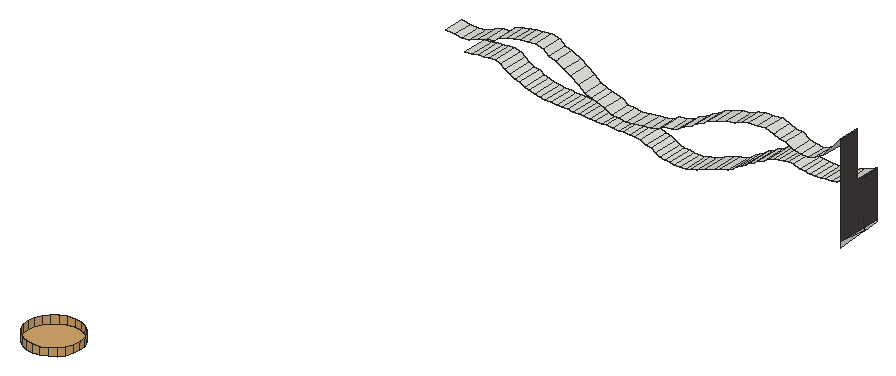
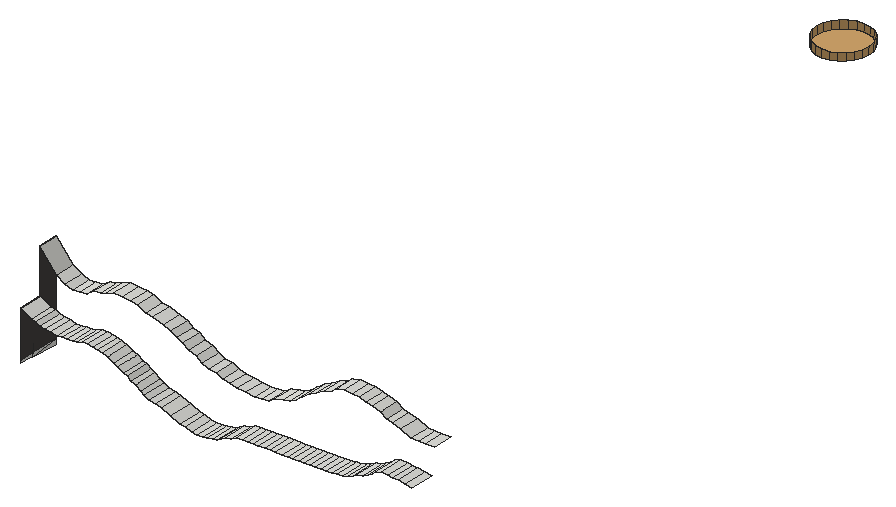
# SketchUp Ruby script. Lengths in inches.
U = 1.inch
M = Sketchup.active_model
def pt(a) = Geom::Point3d.new(a.map { |v| v * U })
def face(e, loops, mat)
  f = e.add_face(loops[0].map { |a| pt(a) })
  loops[1..].each { |l| e.add_face(l.map { |a| pt(a) }).erase! }
  f.material = f.back_material = mat if mat
  f
end
# faces: each face lists its corners as indices into pts; further lists are holes
def faces(e, pts, list, mat = nil) = list.each { |f| face(e, (f[0].is_a?(Array) ? f : [f]).map { |l| l.map { |i| pts[i] } }, mat) }
# xy, xz, yz: faces in a plane at the given z, y or x. An outline is a flat list of corners, or four numbers for a rectangle; further outlines are holes
def ring(l) = l.size == 4 ? [[l[0], l[1]], [l[2], l[1]], [l[2], l[3]], [l[0], l[3]]] : l.each_slice(2).to_a
def flat(e, list, mat, &to3) = list.each { |f| face(e, (f[0].is_a?(Array) ? f : [f]).map { |l| ring(l).map { |u, v| to3.(u, v) } }, mat) }
def xy(e, z, list, mat = nil) = flat(e, list, mat) { |x, y| [x, y, z] }
def xz(e, y, list, mat = nil) = flat(e, list, mat) { |x, z| [x, y, z] }
def yz(e, x, list, mat = nil) = flat(e, list, mat) { |y, z| [x, y, z] }
def lines(e, pts, list) = list.each { |a, b| e.add_line(pt(pts[a]), pt(pts[b])) }
# prism: a flat outline (further loops are holes) pulled along v
def prism(e, loops, v, mat = nil)
  f = face(e, loops, mat); d = Geom::Vector3d.new(v.map { |x| x * U })
  f.pushpull(f.normal.samedirection?(d) ? d.length : -d.length)
end
def box(e, o, s, mat = nil) = prism(e, [[o, [o[0] + s[0], o[1], o[2]], [o[0] + s[0], o[1] + s[1], o[2]], [o[0], o[1] + s[1], o[2]]]], [0, 0, s[2]], mat)
def at(x, y, z, deg = 0) = Geom::Transformation.translation(pt([x, y, z])) * Geom::Transformation.rotation(ORIGIN, Z_AXIS, deg.degrees)
def axes(o, x, y, z) = Geom::Transformation.new([*x, 0, *y, 0, *z, 0, *pt(o).to_a, 1])
def part(name) = M.definitions.add(name)
# library, detail: a bought-in or finely detailed component or shape, given as its bounding box
def library(name, o, s) = part(name).tap { |d| box(d.entities, o, s) }
def detail(e, o, s) = box(e.add_group.entities, o, s)
def put(e, d, t, mat = nil) = e.add_instance(d, t).tap { |i| i.material = mat if mat }
def group(e, t, mat = nil) = e.add_group.tap { |g| g.transformation = t; g.material = mat if mat }.entities
root = M.entities
M.materials.add("[Field Square Tile]").color = [211, 167, 108]
M.materials.add("[Granite Tile]1").color = [68, 65, 63]
xy(root,250.6875,[[3013.293,2328.207,3012.581,2328.3,3011.918,2328.575,3011.348,2329.012,3010.911,2329.582,3010.636,2330.245,3010.543,2330.957,3010.636,2331.668,3010.911,2332.332,3011.348,2332.901,3011.918,2333.338,3012.581,2333.613,3013.293,2333.707,3014.004,2333.613,3014.668,2333.338,3015.237,2332.901,3015.674,2332.332,3015.949,2331.668,3016.043,2330.957,3015.949,2330.245,3015.674,2329.582,3015.237,2329.012,3014.668,2328.575,3014.004,2328.3]],"[Field Square Tile]")
yz(root,3043.095,[[2396.678,240.932,2396.678,241.519,2399.776,241.17],[2399.81,241.167,2399.776,241.17,2399.809,241.173],[2399.776,241.17,2396.678,241.519,2399.769,241.519,2399.809,241.173],[2399.809,241.173,2399.769,241.519,2401.365,241.519,2401.365,241.293]])
yz(root,3043.095,[[2396.678,241.519,2396.678,251.165,2398.803,251.165,2398.803,246.426,2401.365,246.426,2401.365,241.519]],"[Granite Tile]1")
p = [[3023.517,2398.803,241.17],[3023.517,2401.365,241.17],[3023.987,2401.365,241.121],[3023.987,2398.803,241.121],[3024.593,2401.365,241.09],[3024.593,2398.803,241.09],
  [3025.16,2401.365,241.138],[3025.16,2398.803,241.138],[3025.8,2401.365,241.346],[3025.8,2398.803,241.346],[3022.519,2398.803,241.332],[3022.519,2401.365,241.332],
  [3022.987,2401.365,241.243],[3022.987,2398.803,241.243],[3022.1,2398.803,241.566],[3022.1,2401.365,241.566],[3026.391,2401.365,241.456],[3026.391,2398.803,241.456],
  [3027.326,2401.365,241.847],[3027.326,2398.803,241.847],[3021.594,2398.803,241.837],[3021.594,2401.365,241.837],[3021.021,2398.803,241.967],[3021.021,2401.365,241.967],
  [3028.331,2401.365,242.229],[3028.331,2398.803,242.229],[3020.44,2398.803,242.199],[3020.44,2401.365,242.199],[3019.814,2398.803,242.277],[3019.814,2401.365,242.277],
  [3028.892,2401.365,242.424],[3028.892,2398.803,242.424],[3013.967,2398.803,242.35],[3013.967,2401.365,242.35],[3014.549,2401.365,242.342],[3014.549,2398.803,242.342],
  [3015.131,2401.365,242.334],[3015.131,2398.803,242.334],[3015.713,2401.365,242.326],[3015.713,2398.803,242.326],[3016.433,2401.365,242.317],[3016.433,2398.803,242.317],
  [3016.903,2401.365,242.312],[3016.903,2398.803,242.312],[3017.544,2401.365,242.304],[3017.544,2398.803,242.304],[3018.208,2401.365,242.296],[3018.208,2398.803,242.296],
  [3018.66,2401.365,242.291],[3018.66,2398.803,242.291],[3019.298,2401.365,242.283],[3019.298,2398.803,242.283],[3010.485,2398.803,242.466],[3010.485,2401.365,242.466],
  [3011.061,2401.365,242.428],[3011.061,2398.803,242.428],[3011.64,2401.365,242.403],[3011.64,2398.803,242.403],[3012.22,2401.365,242.385],[3012.22,2398.803,242.385],
  [3012.802,2401.365,242.371],[3012.802,2398.803,242.371],[3013.384,2401.365,242.36],[3013.384,2398.803,242.36],[3029.61,2401.365,242.605],[3029.61,2398.803,242.605],
  [3009.357,2398.803,242.599],[3009.357,2401.365,242.599],[3009.917,2401.365,242.518],[3009.917,2398.803,242.518],[3008.804,2398.803,242.75],[3008.804,2401.365,242.75],
  [3030.123,2401.365,242.907],[3030.123,2398.803,242.907],[3008.316,2398.803,242.921],[3008.316,2401.365,242.921],[3007.825,2398.803,243.216],[3007.825,2401.365,243.216],
  [3030.495,2401.365,243.144],[3030.495,2398.803,243.144],[3031.044,2401.365,243.516],[3031.044,2398.803,243.516],[3007.277,2398.803,243.332],[3007.277,2401.365,243.332],
  [3006.732,2398.803,243.589],[3006.732,2401.365,243.589],[3031.518,2401.365,243.711],[3031.518,2398.803,243.711],[3006.251,2398.803,243.88],[3006.251,2401.365,243.88],
  [3031.849,2401.365,244.02],[3031.849,2398.803,244.02],[3005.874,2398.803,244.194],[3005.874,2401.365,244.194],[3002.086,2398.803,243.992],[3002.086,2401.365,243.992],
  [3002.789,2401.365,244.076],[3002.789,2398.803,244.076],[3032.293,2401.365,244.206],[3032.293,2398.803,244.206],[3003.488,2401.365,244.207],[3003.488,2398.803,244.207],
  [3004.073,2401.365,244.266],[3004.073,2398.803,244.266],[3005.277,2398.803,244.387],[3005.277,2401.365,244.387],[3032.882,2401.365,244.569],[3032.882,2398.803,244.569],
  [3004.614,2401.365,244.296],[3004.614,2398.803,244.296],[3033.352,2401.365,244.757],[3033.352,2398.803,244.757],[3033.969,2401.365,245.125],[3033.969,2398.803,245.125],
  [3019.165,2396.678,245.064],[3019.165,2398.803,245.064],[3019.875,2398.803,244.949],[3019.875,2396.678,244.949],[3020.589,2398.803,244.867],[3020.589,2396.678,244.867],
  [3021.495,2398.803,245.007],[3021.495,2396.678,245.007],[3022.439,2398.803,245.121],[3022.439,2396.678,245.121],[3018.452,2396.678,245.459],[3018.452,2398.803,245.459],
  [3023.204,2398.803,245.254],[3023.204,2396.678,245.254],[3034.473,2401.365,245.32],[3034.473,2398.803,245.32],[3038.174,2398.803,245.272],[3038.174,2401.365,245.272],
  [3038.732,2401.365,245.235],[3038.732,2398.803,245.235],[3039.286,2401.365,245.216],[3039.286,2398.803,245.216],[3039.851,2401.365,245.34],[3039.851,2398.803,245.34],
  [3023.956,2398.803,245.41],[3023.956,2396.678,245.41],[3034.955,2401.365,245.411],[3034.955,2398.803,245.411],[3036.521,2398.803,245.552],[3036.521,2401.365,245.552],
  [3037.129,2401.365,245.346],[3037.129,2398.803,245.346],[3037.623,2401.365,245.309],[3037.623,2398.803,245.309],[3040.483,2401.365,245.423],[3040.483,2398.803,245.423],
  [3024.59,2398.803,245.775],[3024.59,2396.678,245.775],[3035.503,2401.365,245.481],[3035.503,2398.803,245.481],[3041.061,2401.365,245.516],[3041.061,2398.803,245.516],
  [3017.577,2396.678,245.671],[3017.577,2398.803,245.671],[3035.985,2401.365,245.59],[3035.985,2398.803,245.59],[3041.441,2401.365,245.763],[3041.441,2398.803,245.763],
  [3016.902,2396.678,245.834],[3016.902,2398.803,245.834],[3016.314,2396.678,246.129],[3016.314,2398.803,246.129],[3025.386,2398.803,245.88],[3025.386,2396.678,245.88],
  [3041.91,2401.365,245.896],[3041.91,2398.803,245.896],[3026.099,2398.803,246.16],[3026.099,2396.678,246.16],[3043.095,2401.365,246.426],[3043.095,2398.803,246.426],
  [3015.683,2396.678,246.633],[3015.683,2398.803,246.633],[3026.696,2398.803,246.573],[3026.696,2396.678,246.573],[3014.869,2396.678,247.185],[3014.869,2398.803,247.185],
  [3027.486,2398.803,246.902],[3027.486,2396.678,246.902],[3002.692,2396.678,246.79],[3002.692,2398.803,246.79],[3003.471,2398.803,246.747],[3003.471,2396.678,246.747],
  [3004.218,2398.803,246.831],[3004.218,2396.678,246.831],[3001.738,2396.678,246.838],[3001.738,2398.803,246.838],[3005.26,2398.803,247.251],[3005.26,2396.678,247.251],
  [3028.088,2398.803,247.347],[3028.088,2396.678,247.347],[3014.157,2396.678,247.553],[3014.157,2398.803,247.553],[3006.134,2398.803,247.546],[3006.134,2396.678,247.546],
  [3028.762,2398.803,247.615],[3028.762,2396.678,247.615],[3006.796,2398.803,247.657],[3006.796,2396.678,247.657],[3013.266,2396.678,248.059],[3013.266,2398.803,248.059],
  [3029.349,2398.803,248.057],[3029.349,2396.678,248.057],[3007.429,2398.803,248.162],[3007.429,2396.678,248.162],[3012.575,2396.678,248.257],[3012.575,2398.803,248.257],
  [3030.114,2398.803,248.322],[3030.114,2396.678,248.322],[3008.223,2398.803,248.408],[3008.223,2396.678,248.408],[3038.911,2396.678,248.295],[3038.911,2398.803,248.295],
  [3039.62,2398.803,248.218],[3039.62,2396.678,248.218],[3040.437,2398.803,248.558],[3040.437,2396.678,248.558],[3012.044,2396.678,248.687],[3012.044,2398.803,248.687],
  [3031.225,2398.803,248.655],[3031.225,2396.678,248.655],[3038.2,2396.678,248.42],[3038.2,2398.803,248.42],[3008.922,2398.803,248.521],[3008.922,2396.678,248.521],
  [3037.403,2396.678,248.895],[3037.403,2398.803,248.895],[3009.616,2398.803,248.723],[3009.616,2396.678,248.723],[3041.372,2398.803,249.022],[3041.372,2396.678,249.022],
  [3010.315,2398.803,248.801],[3010.315,2396.678,248.801],[3011.212,2396.678,248.851],[3011.212,2398.803,248.851],[3031.998,2398.803,248.795],[3031.998,2396.678,248.795],
  [3032.861,2398.803,249.194],[3032.861,2396.678,249.194],[3036.699,2396.678,248.962],[3036.699,2398.803,248.962],[3036.06,2396.678,249.206],[3036.06,2398.803,249.206],
  [3043.095,2398.803,251.165],[3043.095,2396.678,251.165],[3033.534,2398.803,249.323],[3033.534,2396.678,249.323],[3035.315,2396.678,249.478],[3035.315,2398.803,249.478],
  [3034.457,2398.803,249.406],[3034.457,2396.678,249.406],[3013.293,2328.207,251.5],[3012.581,2328.3,251.5],[3012.581,2328.3,250.6875],[3013.293,2328.207,250.6875],
  [3014.004,2328.3,251.5],[3014.004,2328.3,250.6875],[3011.918,2328.575,251.5],[3011.918,2328.575,250.6875],[3014.668,2328.575,251.5],[3014.668,2328.575,250.6875],
  [3011.348,2329.012,251.5],[3011.348,2329.012,250.6875],[3015.237,2329.012,251.5],[3015.237,2329.012,250.6875],[3010.911,2329.582,251.5],[3010.911,2329.582,250.6875],
  [3015.674,2329.582,251.5],[3015.674,2329.582,250.6875],[3010.636,2330.245,251.5],[3010.636,2330.245,250.6875],[3015.949,2330.245,251.5],[3015.949,2330.245,250.6875],
  [3010.543,2330.957,251.5],[3010.543,2330.957,250.6875],[3016.043,2330.957,251.5],[3016.043,2330.957,250.6875],[3010.636,2331.668,251.5],[3010.636,2331.668,250.6875],
  [3015.949,2331.668,251.5],[3015.949,2331.668,250.6875],[3010.911,2332.332,251.5],[3010.911,2332.332,250.6875],[3015.674,2332.332,251.5],[3015.674,2332.332,250.6875],
  [3011.348,2332.901,251.5],[3011.348,2332.901,250.6875],[3015.237,2332.901,251.5],[3015.237,2332.901,250.6875],[3011.918,2333.338,251.5],[3011.918,2333.338,250.6875],
  [3014.668,2333.338,251.5],[3014.668,2333.338,250.6875],[3012.581,2333.613,251.5],[3012.581,2333.613,250.6875],[3014.004,2333.613,251.5],[3014.004,2333.613,250.6875],
  [3013.293,2333.707,251.5],[3013.293,2333.707,250.6875],[3043.095,2400.588,246.171],[3043.095,2399.573,246.265],[3043.095,2401.365,246.273],[3043.095,2399.769,241.519],
  [3043.095,2399.667,242.384]]
faces(root,p,[[0,1,2,3],[3,2,4,5],[5,4,6,7],[7,6,8,9],[10,11,12,13],[13,12,1,0],[14,15,11,10],[9,8,16,17],
  [17,16,18,19],[20,21,15,14],[22,23,21,20],[19,18,24,25],[26,27,23,22],[28,29,27,26],[25,24,30,31],[32,33,34,35],
  [35,34,36,37],[37,36,38,39],[39,38,40,41],[41,40,42,43],[43,42,44,45],[45,44,46,47],[47,46,48,49],[49,48,50,51],
  [51,50,29,28],[52,53,54,55],[55,54,56,57],[57,56,58,59],[59,58,60,61],[61,60,62,63],[63,62,33,32],[31,30,64,65],
  [66,67,68,69],[69,68,53,52],[70,71,67,66],[65,64,72,73],[74,75,71,70],[76,77,75,74],[73,72,78,79],[79,78,80,81],
  [82,83,77,76],[84,85,83,82],[81,80,86,87],[88,89,85,84],[87,86,90,91],[92,93,89,88],[94,95,96,97],[91,90,98,99],
  [97,96,100,101],[101,100,102,103],[104,105,93,92],[99,98,106,107],[103,102,108,109],[109,108,105,104],[107,106,110,111],[111,110,112,113],
  [114,115,116,117],[117,116,118,119],[119,118,120,121],[121,120,122,123],[124,125,115,114],[123,122,126,127],[113,112,128,129],[130,131,132,133],
  [133,132,134,135],[135,134,136,137],[127,126,138,139],[129,128,140,141],[142,143,144,145],[145,144,146,147],[147,146,131,130],[137,136,148,149],
  [139,138,150,151],[141,140,152,153],[149,148,154,155],[156,157,125,124],[153,152,158,159],[155,154,160,161],[159,158,143,142],[162,163,157,156],
  [164,165,163,162],[151,150,166,167],[161,160,168,169],[167,166,170,171],[169,168,172,173],[174,175,165,164],[171,170,176,177],[178,179,175,174],
  [177,176,180,181],[182,183,184,185],[185,184,186,187],[188,189,183,182],[187,186,190,191],[181,180,192,193],[194,195,179,178],[191,190,196,197],
  [193,192,198,199],[197,196,200,201],[202,203,195,194],[199,198,204,205],[201,200,206,207],[208,209,203,202],[205,204,210,211],[207,206,212,213],
  [214,215,216,217],[217,216,218,219],[220,221,209,208],[211,210,222,223],[224,225,215,214],[213,212,226,227],[228,229,225,224],[227,226,230,231],
  [219,218,232,233],[231,230,234,235],[236,237,221,220],[223,222,238,239],[235,234,237,236],[239,238,240,241],[242,243,229,228],[244,245,243,242],
  [233,232,246,247],[241,240,248,249],[250,251,245,244],[249,248,252,253],[253,252,251,250]])
faces(root,p,[[254,255,256,257],[258,254,257,259],[255,260,261,256],[262,258,259,263],[260,264,265,261],[266,262,263,267],[264,268,269,265],[270,266,267,271],
  [268,272,273,269],[274,270,271,275],[272,276,277,273],[278,274,275,279],[276,280,281,277],[282,278,279,283],[280,284,285,281],[286,282,283,287],
  [284,288,289,285],[290,286,287,291],[288,292,293,289],[294,290,291,295],[292,296,297,293],[298,294,295,299],[296,300,301,297],[300,298,299,301]],"[Field Square Tile]")
lines(root,p,[[302,303],[304,302],[305,306]])
